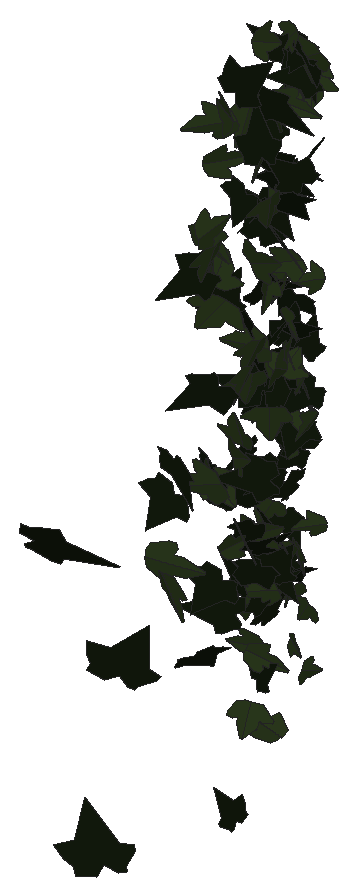
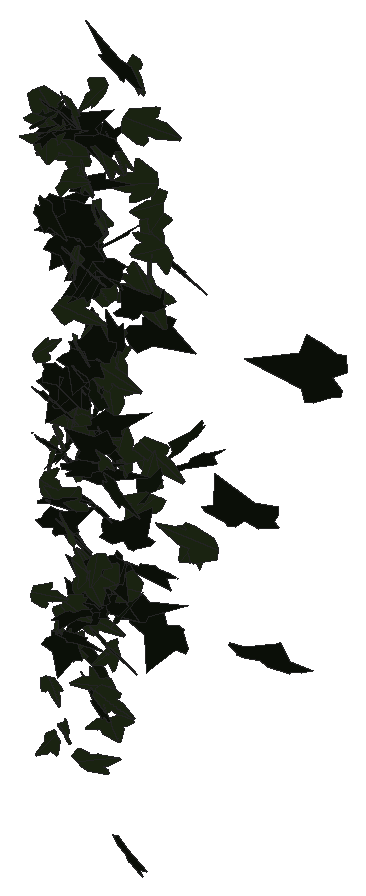
# SketchUp Ruby script. Lengths in inches.
U = 1.inch
M = Sketchup.active_model
def pt(a) = Geom::Point3d.new(a.map { |v| v * U })
def face(e, loops, mat)
  f = e.add_face(loops[0].map { |a| pt(a) })
  loops[1..].each { |l| e.add_face(l.map { |a| pt(a) }).erase! }
  f.material = f.back_material = mat if mat
  f
end
# faces: each face lists its corners as indices into pts; further lists are holes
def faces(e, pts, list, mat = nil) = list.each { |f| face(e, (f[0].is_a?(Array) ? f : [f]).map { |l| l.map { |i| pts[i] } }, mat) }
# xy, xz, yz: faces in a plane at the given z, y or x. An outline is a flat list of corners, or four numbers for a rectangle; further outlines are holes
def ring(l) = l.size == 4 ? [[l[0], l[1]], [l[2], l[1]], [l[2], l[3]], [l[0], l[3]]] : l.each_slice(2).to_a
def flat(e, list, mat, &to3) = list.each { |f| face(e, (f[0].is_a?(Array) ? f : [f]).map { |l| ring(l).map { |u, v| to3.(u, v) } }, mat) }
def xy(e, z, list, mat = nil) = flat(e, list, mat) { |x, y| [x, y, z] }
def xz(e, y, list, mat = nil) = flat(e, list, mat) { |x, z| [x, y, z] }
def yz(e, x, list, mat = nil) = flat(e, list, mat) { |y, z| [x, y, z] }
def lines(e, pts, list) = list.each { |a, b| e.add_line(pt(pts[a]), pt(pts[b])) }
# prism: a flat outline (further loops are holes) pulled along v
def prism(e, loops, v, mat = nil)
  f = face(e, loops, mat); d = Geom::Vector3d.new(v.map { |x| x * U })
  f.pushpull(f.normal.samedirection?(d) ? d.length : -d.length)
end
def box(e, o, s, mat = nil) = prism(e, [[o, [o[0] + s[0], o[1], o[2]], [o[0] + s[0], o[1] + s[1], o[2]], [o[0], o[1] + s[1], o[2]]]], [0, 0, s[2]], mat)
def at(x, y, z, deg = 0) = Geom::Transformation.translation(pt([x, y, z])) * Geom::Transformation.rotation(ORIGIN, Z_AXIS, deg.degrees)
def axes(o, x, y, z) = Geom::Transformation.new([*x, 0, *y, 0, *z, 0, *pt(o).to_a, 1])
def part(name) = M.definitions.add(name)
# library, detail: a bought-in or finely detailed component or shape, given as its bounding box
def library(name, o, s) = part(name).tap { |d| box(d.entities, o, s) }
def detail(e, o, s) = box(e.add_group.entities, o, s)
def put(e, d, t, mat = nil) = e.add_instance(d, t).tap { |i| i.material = mat if mat }
def group(e, t, mat = nil) = e.add_group.tap { |g| g.transformation = t; g.material = mat if mat }.entities
root = M.entities
M.materials.add("1026 AP 7946 SUNNY SIDE UP").color = [254, 231, 186]
M.materials.add("efeu1").color = [18, 25, 13]
M.materials.add("efeu2").color = [43, 57, 29]
c1 = part("ivyleaf_9")
p = [[1.54,2.16,1.25],[1.36,2.04,1.19],[-0.21,0.99,0.68],[-0.71,1.11,0.82],[-0.85,0.86,0.67],[-0.8,0.17,0.21],
  [-0.9,-0.01,0.1],[-0.67,-0.16,-0.02],[-0.08,-0.08,-0.05],[-0.03,-0.6,-0.4],[0.65,-0.88,-0.66],[0.83,-0.6,-0.49],
  [1.29,-0.42,-0.43],[1.8125,-0.07,-0.26],[1.21,0.44,0.15]]
faces(c1.entities,p,[[0,1,2,3,4,5,6,7,8,9,10,11,12,13,14]],"efeu1")
c2 = part("ivyleaf_10")
p = [[0,0.5,-0.03],[-0.0625,2.02,-0.43],[-0.19,2.01,-0.46],[-0.54,1.05,-0.29],[-0.52,0.625,-0.18],[-0.83,0.76,-0.28],
  [-1.16,0.64,-0.33],[-1.15,0.33,-0.24],[-0.77,-0.39,0.02],[-0.3,-0.51,0.16],[0.04,-0.48,0.23],[-0.02,2.01,-0.4375],
  [-0.06,2.01,-0.43],[0.04,-0.49,0.23],[0.67,-0.49,0.14],[1.38,0.36,-0.2],[1.375,0.51,-0.24],[0.81,0.65,-0.19],
  [0.62,0.59,-0.15],[0.6,1.09,-0.28],[0.5,1.23,-0.31]]
faces(c2.entities,p,[[0,1,2,3,4,5,6,7,8,9,10],[11,12,0,13,14,15,16,17,18,19,20]],"efeu2")
put(root,c1,axes([143.91,204.23,258.27],[0.4442,-0.05472,0.34587],[0.52307,-0.04862,-0.29654],[0.114,0.43631,0.01296]),"1026 AP 7946 SUNNY SIDE UP")
put(root,c1,axes([145.62,204.32,250.95],[-0.6745,-0.03704,0.05582],[0.07961,0.04334,0.44203],[-0.06609,0.43022,-0.03716]),"1026 AP 7946 SUNNY SIDE UP")
put(root,c1,axes([145.2,205.4375,254.96],[-0.43099,0.00527,0.31558],[0.47929,-0.0364,0.28143],[0.04816,0.40942,0.02338]),"1026 AP 7946 SUNNY SIDE UP")
put(root,c2,axes([144.47,208,255.81],[-0.41617,0.22329,-0.15177],[0.14377,-0.12113,-0.35602],[-0.39647,-0.27831,0.03021]),"1026 AP 7946 SUNNY SIDE UP")
put(root,c1,axes([144.38,208.25,257.83],[-0.24288,-0.27765,0.15078],[-0.09553,-0.13538,-0.32789],[0.48537,-0.16558,0.01091]),"1026 AP 7946 SUNNY SIDE UP")
put(root,c1,axes([145.43,208.44,260.77],[0.0087,0.02505,-0.3572],[-0.09637,-0.34142,-0.02841],[-0.53829,0.06153,-0.00069]),"1026 AP 7946 SUNNY SIDE UP")
put(root,c1,axes([144.24,208.49,258.49],[0.14987,-0.32445,0.08732],[0.03251,-0.08418,-0.34884],[0.52702,0.09746,-0.00331]),"1026 AP 7946 SUNNY SIDE UP")
put(root,c2,axes([143.93,208.34,256.05],[0.03397,-0.0484,-0.39616],[0.59854,-0.06837,0.03052],[-0.11239,-0.37876,0.04279]),"1026 AP 7946 SUNNY SIDE UP")
put(root,c2,axes([145.09,208.79,258.1],[-0.27734,0.02978,0.32535],[-0.49487,-0.06011,-0.17568],[0.06026,-0.35655,0.05463]),"1026 AP 7946 SUNNY SIDE UP")
put(root,c1,axes([144.78,208.55,253.875],[0.2302,0.31567,0.08074],[0.05949,0.06686,-0.35802],[-0.50728,0.15109,-0.00535]),"1026 AP 7946 SUNNY SIDE UP")
put(root,c2,axes([144.91,208.93,263.68],[0.00073,-0.39232,0.02905],[0.0109,-0.03041,-0.40428],[0.61863,0.001,0.00709]),"1026 AP 7946 SUNNY SIDE UP")
put(root,c1,axes([144.71,208.98,263.08],[-0.58845,0.09659,-0.02919],[0.02876,-0.04412,-0.3965],[-0.15589,-0.37275,0.03701]),"1026 AP 7946 SUNNY SIDE UP")
put(root,c1,axes([144.96,209.17,255.52],[-0.45271,-0.12464,-0.02536],[0.05178,-0.01612,-0.32203],[0.19272,-0.28845,0.02695]),"1026 AP 7946 SUNNY SIDE UP")
put(root,c2,axes([145.35,208.93,267.17],[0.05949,-0.05854,-0.35999],[-0.25234,0.3101,-0.06968],[0.49611,0.16475,0.00773]),"1026 AP 7946 SUNNY SIDE UP")
put(root,c2,axes([144.75,208.85,264.1],[0.03865,0.05038,-0.38805],[0.18583,0.35804,0.05933],[0.5684,-0.12048,0.00699]),"1026 AP 7946 SUNNY SIDE UP")
put(root,c2,axes([144.74,209.2,257.73],[-0.37546,0.20756,-0.02116],[-0.00703,0.02791,0.32557],[0.32808,0.23814,-0.01724]),"1026 AP 7946 SUNNY SIDE UP")
put(root,c2,axes([144.84,209.28,262.18],[0.51569,0.08418,-0.16296],[-0.2691,0.04622,-0.3389],[-0.0857,0.36138,0.08357]),"1026 AP 7946 SUNNY SIDE UP")
put(root,c1,axes([145.04,209.48,254.58],[-0.21895,-0.02923,0.30761],[-0.4295,-0.12425,-0.1444],[0.19576,-0.3053,0.02722]),"1026 AP 7946 SUNNY SIDE UP")
put(root,c2,axes([144.31,209.66,262.91],[-0.02449,0.05967,0.36681],[0.3821,-0.26139,0.0546],[0.41913,0.24178,-0.02834]),"1026 AP 7946 SUNNY SIDE UP")
put(root,c2,axes([145.34,209.58,260.57],[0.06103,-0.33213,0.12291],[0.04565,-0.11852,-0.34487],[0.55405,0.04635,0.01488]),"1026 AP 7946 SUNNY SIDE UP")
put(root,c2,axes([144.67,209.6875,266.47],[-0.1374,-0.08334,0.35157],[-0.32061,-0.27493,-0.12439],[0.45069,-0.22098,0.01869]),"1026 AP 7946 SUNNY SIDE UP")
put(root,c1,axes([144.26,209.76,257.83],[0.0974,-0.24531,0.18824],[0.06358,-0.17966,-0.26167],[0.47807,0.07387,-0.00355]),"1026 AP 7946 SUNNY SIDE UP")
put(root,c2,axes([144.14,209.625,263.62],[-0.35989,0.05646,-0.24104],[0.33274,-0.10756,-0.24029],[-0.18137,-0.30937,0.03747]),"1026 AP 7946 SUNNY SIDE UP")
put(root,c1,axes([145.09,209.58,267.42],[-0.19331,0.22963,0.3027],[0.26332,-0.24091,0.26591],[0.52212,0.20652,-0.02204]),"1026 AP 7946 SUNNY SIDE UP")
put(root,c1,axes([144.625,209.54,261.95],[-0.23618,-0.0729,0.29027],[0.39041,0.13422,0.17266],[-0.23996,0.29012,-0.00478]),"1026 AP 7946 SUNNY SIDE UP")
put(root,c2,axes([144.86,209.8,258.22],[-0.21327,0.10122,0.26268],[0.36849,-0.10391,0.17069],[0.22264,0.26893,-0.03088]),"1026 AP 7946 SUNNY SIDE UP")
put(root,c2,axes([144.48,209.64,262.59],[0.50208,-0.04558,-0.03787],[0.06494,0.03285,0.33014],[-0.06491,-0.3197,0.0374]),"1026 AP 7946 SUNNY SIDE UP")
put(root,c2,axes([145.41,209.83,261.17],[-0.04986,-0.34863,0.07419],[0.00198,-0.0744,-0.36099],[0.5604,-0.03076,0.00787]),"1026 AP 7946 SUNNY SIDE UP")
put(root,c1,axes([145.63,209.96,257.88],[-0.31775,-0.05214,0.25719],[-0.36035,-0.1035,-0.21373],[0.17702,-0.3043,0.02659]),"1026 AP 7946 SUNNY SIDE UP")
put(root,c2,axes([144.32,209.68,257.5625],[0.20932,0.25762,0.17923],[0.14155,0.14754,-0.29767],[-0.46651,0.16036,-0.0099]),"1026 AP 7946 SUNNY SIDE UP")
put(root,c2,axes([145.16,209.91,252.1],[0.32918,0.21096,-0.08231],[-0.06538,-0.0727,-0.30584],[-0.34931,0.21241,-0.02032]),"1026 AP 7946 SUNNY SIDE UP")
put(root,c2,axes([144.91,209.91,258.64],[-0.45055,0.09748,-0.03646],[-0.03966,0.03701,0.3108],[0.15847,0.2864,-0.02586]),"1026 AP 7946 SUNNY SIDE UP")
put(root,c2,axes([145.11,210.03,260.17],[-0.21876,-0.31771,-0.00263],[0.00896,-0.00168,-0.35727],[0.49949,-0.13912,0.00526]),"1026 AP 7946 SUNNY SIDE UP")
put(root,c2,axes([144.26,209.85,265.23],[0.03853,-0.07058,0.36115],[0.13044,0.34334,0.06717],[-0.54759,0.07682,0.04141]),"1026 AP 7946 SUNNY SIDE UP")
put(root,c1,axes([145.41,210.02,265.79],[-0.27882,-0.20444,0.27],[0.22964,0.22038,0.27894],[-0.47111,0.22842,-0.02383]),"1026 AP 7946 SUNNY SIDE UP")
put(root,c1,axes([144.65,210.35,261.39],[0.01829,-0.05422,0.30423],[0.09296,-0.28965,-0.05882],[0.46335,0.06025,-0.00021]),"1026 AP 7946 SUNNY SIDE UP")
put(root,c1,axes([144.53,210.25,256.8125],[0.22077,0.05238,0.2677],[-0.41191,-0.01538,0.14909],[0.06074,-0.2947,0.03802]),"1026 AP 7946 SUNNY SIDE UP")
put(root,c1,axes([144.72,210.23,254.875],[-0.03217,-0.25559,0.12409],[0.01082,0.12174,0.26485],[-0.44514,0.02143,-0.00253]),"1026 AP 7946 SUNNY SIDE UP")
put(root,c1,axes([144.67,210.03,249.17],[-0.05881,0.12042,0.27808],[-0.18278,0.24342,-0.12736],[-0.42625,-0.12099,0.01625]),"1026 AP 7946 SUNNY SIDE UP")
put(root,c1,axes([145.07,210.39,255.33],[0.02992,0.04935,-0.28548],[-0.07371,-0.2736,-0.05506],[-0.43685,0.04954,-0.01027]),"1026 AP 7946 SUNNY SIDE UP")
put(root,c1,axes([144.66,210.24,256.125],[0.33555,-0.11392,-0.1911],[-0.27399,0.0648,-0.24799],[0.20372,0.27479,-0.01877]),"1026 AP 7946 SUNNY SIDE UP")
put(root,c1,axes([145.01,210.4,252.57],[-0.06046,0.14227,0.23716],[0.11682,-0.21719,0.15032],[0.40806,0.08326,-0.0079]),"1026 AP 7946 SUNNY SIDE UP")
put(root,c2,axes([144.375,210.18,255.64],[-0.00582,-0.13898,0.26939],[0.06303,0.25967,0.14385],[-0.46247,0.03714,0.01622]),"1026 AP 7946 SUNNY SIDE UP")
put(root,c2,axes([145.07,210.39,260.78],[-0.12277,0.02895,0.35175],[-0.52892,-0.07238,-0.07338],[0.10139,-0.34253,0.04313]),"1026 AP 7946 SUNNY SIDE UP")
put(root,c1,axes([144.77,210.45,258.125],[-0.33274,0.15016,-0.12778],[0.12346,-0.1032,-0.26548],[-0.28119,-0.223,0.03465]),"1026 AP 7946 SUNNY SIDE UP")
put(root,c2,axes([144.97,210.32,253.2],[0.09614,0.04851,0.27505],[0.37204,0.1239,-0.07837],[-0.20805,0.24397,-0.01304]),"1026 AP 7946 SUNNY SIDE UP")
put(root,c2,axes([145.34,210.4,259.23],[-0.36009,-0.24597,-0.00627],[0.04484,-0.02018,-0.3445],[0.38423,-0.22816,0.03433]),"1026 AP 7946 SUNNY SIDE UP")
put(root,c2,axes([144.58,210.5,266.28],[0.44207,-0.2163,0.07976],[0.07273,-0.06853,-0.36489],[0.35452,0.28378,-0.0246]),"1026 AP 7946 SUNNY SIDE UP")
put(root,c2,axes([145.24,210.51,254.8],[-0.17451,-0.00987,0.26233],[-0.32796,-0.15615,-0.10078],[0.23036,-0.22979,0.05525]),"1026 AP 7946 SUNNY SIDE UP")
put(root,c1,axes([144.46,210.66,264.18],[-0.12344,-0.25181,0.14691],[-0.03493,-0.14356,-0.27187],[0.45481,-0.07937,0.01899]),"1026 AP 7946 SUNNY SIDE UP")
put(root,c1,axes([144.875,210.61,259.49],[-0.10681,0.00981,0.31975],[-0.44259,-0.13602,-0.05984],[0.20605,-0.28708,0.03722]),"1026 AP 7946 SUNNY SIDE UP")
put(root,c2,axes([144.83,210.53,262.67],[-0.3099,0.05947,0.29271],[0.44443,-0.03718,0.21002],[0.10174,0.34351,-0.02585]),"1026 AP 7946 SUNNY SIDE UP")
put(root,c2,axes([145.33,210.52,251.34],[0.17042,0.13198,0.23391],[-0.31625,-0.11501,0.16766],[0.26397,-0.22301,0.04986]),"1026 AP 7946 SUNNY SIDE UP")
put(root,c1,axes([144.84,210.5,256.23],[0.09736,0.17611,-0.21135],[-0.08379,-0.19943,-0.19317],[-0.41802,0.08099,-0.01051]),"1026 AP 7946 SUNNY SIDE UP")
put(root,c2,axes([145.23,210.5,264.33],[-0.09107,-0.35462,-0.06145],[0.03312,0.05493,-0.36965],[0.56395,-0.06049,0.01178]),"1026 AP 7946 SUNNY SIDE UP")
put(root,c1,axes([144.97,210.59,254.52],[-0.42206,0.14929,-0.03261],[0.02407,-0.0391,-0.31545],[-0.23903,-0.26754,0.02582]),"1026 AP 7946 SUNNY SIDE UP")
put(root,c1,axes([145.26,210.66,257.72],[-0.42536,0.03262,-0.06889],[0.09739,-0.04223,-0.27882],[-0.06529,-0.27548,0.03291]),"1026 AP 7946 SUNNY SIDE UP")
put(root,c1,axes([144.83,210.8125,260.05],[-0.05806,0.00026,0.32225],[-0.08682,-0.31003,-0.00826],[0.48412,-0.05557,0.03716]),"1026 AP 7946 SUNNY SIDE UP")
put(root,c2,axes([144.78,210.64,255.96],[-0.34347,-0.04192,0.22775],[0.34149,0.04258,0.22938],[-0.09395,0.30802,0.00115]),"1026 AP 7946 SUNNY SIDE UP")
put(root,c1,axes([144.79,210.57,255.61],[0.28361,0.24066,-0.01448],[-0.0092,0.02362,0.30936],[0.37908,-0.17948,0.01834]),"1026 AP 7946 SUNNY SIDE UP")
put(root,c1,axes([144.86,210.52,259.07],[-0.03731,0.09049,0.28187],[-0.16403,0.25267,-0.09411],[-0.42159,-0.10631,0.01167]),"1026 AP 7946 SUNNY SIDE UP")
put(root,c2,axes([144.75,210.67,253.18],[0.15918,-0.05165,-0.27939],[-0.39124,0.10736,-0.11625],[0.18704,0.26854,-0.00539]),"1026 AP 7946 SUNNY SIDE UP")
put(root,c2,axes([144.61,210.51,254.25],[-0.01221,-0.05394,-0.30535],[0.13119,0.2842,-0.05393],[0.4547,-0.08345,0.00736]),"1026 AP 7946 SUNNY SIDE UP")
put(root,c1,axes([145.16,210.6875,255.11],[-0.27465,0.08791,0.19696],[0.26677,-0.08705,0.20094],[0.19453,0.2435,0.00251]),"1026 AP 7946 SUNNY SIDE UP")
put(root,c1,axes([144.98,210.63,253.95],[-0.19247,0.27658,-0.0268],[-0.01222,0.02673,0.31172],[0.43688,0.1226,-0.00309]),"1026 AP 7946 SUNNY SIDE UP")
put(root,c2,axes([144.97,211.05,263.96],[-0.00437,0.0136,0.30235],[0.07949,-0.28902,0.0126],[0.45496,0.05063,0.0007]),"1026 AP 7946 SUNNY SIDE UP")
put(root,c2,axes([144.9,210.95,262.05],[0.00015,0.26309,-0.20274],[-0.04986,-0.19737,-0.27093],[-0.51562,0.01916,0.02614]),"1026 AP 7946 SUNNY SIDE UP")
put(root,c1,axes([144.8125,210.77,266.62],[0.00586,-0.02157,-0.35076],[0.38581,0.23657,-0.01129],[0.37244,-0.24472,0.01722]),"1026 AP 7946 SUNNY SIDE UP")
put(root,c1,axes([144.89,211.02,264.02],[-0.30432,0.22318,-0.19083],[0.14337,-0.16618,-0.3033],[-0.43428,-0.21125,0.0336]),"1026 AP 7946 SUNNY SIDE UP")
put(root,c2,axes([145.11,211.14,258.67],[0.01949,0.00659,0.27411],[0.21045,-0.23035,-0.00189],[0.36168,0.13368,-0.01367]),"1026 AP 7946 SUNNY SIDE UP")
put(root,c1,axes([145.03,210.91,255.07],[0.05629,-0.18958,-0.19092],[-0.02451,0.1841,-0.19719],[0.41497,0.03659,0.01425]),"1026 AP 7946 SUNNY SIDE UP")
put(root,c2,axes([145.22,210.78,260.13],[-0.01902,-0.17618,-0.2933],[0.04579,0.28225,-0.1802],[0.52311,-0.03111,0.00511]),"1026 AP 7946 SUNNY SIDE UP")
put(root,c1,axes([144.65,211.0625,256.15],[0.24381,-0.20665,0.07047],[0.03743,-0.06882,-0.26564],[0.34081,0.15539,-0.02123]),"1026 AP 7946 SUNNY SIDE UP")
put(root,c2,axes([144.38,211.08,266.34],[0.42145,-0.1183,0.0566],[0.06314,-0.04622,-0.30093],[0.1956,0.26981,-0.02481]),"1026 AP 7946 SUNNY SIDE UP")
put(root,c1,axes([144.61,211.09,261.54],[0.26174,0.18837,0.21342],[-0.23698,-0.14137,0.25769],[0.36959,-0.22405,0.01409]),"1026 AP 7946 SUNNY SIDE UP")
put(root,c1,axes([144.83,210.83,260.51],[-0.17504,0.25519,-0.07292],[-0.02999,0.07043,0.28704],[0.41594,0.11247,-0.00999]),"1026 AP 7946 SUNNY SIDE UP")
put(root,c2,axes([144.51,211.1875,264.99],[0.22361,-0.24269,0.15532],[0.09571,-0.14038,-0.29012],[0.44011,0.15384,-0.01582]),"1026 AP 7946 SUNNY SIDE UP")
put(root,c1,axes([145.55,211.18,264.65],[0.04415,0.06939,0.31023],[-0.43396,-0.12956,0.05658],[0.21729,-0.27285,0.04997]),"1026 AP 7946 SUNNY SIDE UP")
put(root,c1,axes([145.51,211.05,257.28],[-0.3017,0.22862,-0.03871],[0.02206,-0.03892,-0.30736],[-0.36397,-0.19186,0.01346]),"1026 AP 7946 SUNNY SIDE UP")
put(root,c1,axes([145.17,210.92,264.1875],[0.36845,0.22424,0.04542],[0.07357,0.01288,-0.33322],[-0.35134,0.23786,-0.02214]),"1026 AP 7946 SUNNY SIDE UP")
put(root,c2,axes([145.17,211.26,255.45],[-0.07262,-0.18695,0.19795],[-0.05613,-0.19004,-0.19933],[0.41899,-0.05786,0.0076]),"1026 AP 7946 SUNNY SIDE UP")
put(root,c1,axes([144.75,211.09,263.38],[0.47154,-0.19393,-0.09586],[-0.13831,0.03305,-0.36718],[0.30783,0.31192,-0.01814]),"1026 AP 7946 SUNNY SIDE UP")
put(root,c1,axes([144.625,210.97,263.12],[-0.14167,-0.02741,0.32879],[0.42671,0.16991,0.09491],[-0.26806,0.28496,-0.02269]),"1026 AP 7946 SUNNY SIDE UP")
put(root,c2,axes([145.15,211.33,254.51],[0.09874,-0.08801,0.22988],[0.18467,-0.19044,-0.11229],[0.32972,0.13302,-0.00595]),"1026 AP 7946 SUNNY SIDE UP")
put(root,c2,axes([145.08,211.32,260.38],[0.08033,-0.18666,-0.18995],[0.09302,-0.1737,0.19818],[-0.40073,-0.07774,0.00793]),"1026 AP 7946 SUNNY SIDE UP")
put(root,c1,axes([144.47,211.15,263.9],[-0.11946,-0.1463,-0.2863],[0.24585,0.22938,-0.16759],[0.42696,-0.17301,0.0164]),"1026 AP 7946 SUNNY SIDE UP")
put(root,c2,axes([145.25,211.27,262.55],[0.20593,0.03684,-0.28677],[-0.42576,-0.06562,-0.14047],[-0.11812,0.30075,0.00635]),"1026 AP 7946 SUNNY SIDE UP")
put(root,c1,axes([144.74,211.41,265.71],[-0.28344,-0.08501,0.24633],[-0.31454,-0.13384,-0.20475],[0.24671,-0.2683,0.02197]),"1026 AP 7946 SUNNY SIDE UP")
put(root,c2,axes([145.23,211.32,254.375],[-0.24041,-0.12217,-0.15773],[-0.18218,-0.0991,0.20099],[-0.24728,0.19179,0.00526]),"1026 AP 7946 SUNNY SIDE UP")
put(root,c2,axes([144.6,210.98,267.84],[-0.02496,0.12198,0.32132],[-0.07971,0.30708,-0.12486],[-0.51951,-0.05297,0.00372]),"1026 AP 7946 SUNNY SIDE UP")
put(root,c2,axes([144.97,211.41,261.04],[-0.11813,0.09192,-0.24533],[0.20657,-0.19955,-0.12295],[-0.34504,-0.15094,0.01038]),"1026 AP 7946 SUNNY SIDE UP")
put(root,c2,axes([144.59,211.37,256.29],[-0.30579,-0.14849,0.10176],[-0.0949,-0.08404,-0.25091],[0.26466,-0.20169,0.02761]),"1026 AP 7946 SUNNY SIDE UP")
put(root,c2,axes([145.0625,211.23,259.86],[0.34594,0.08814,-0.12978],[0.16522,0.07555,0.24297],[0.17738,-0.24227,0.02681]),"1026 AP 7946 SUNNY SIDE UP")
put(root,c1,axes([144.84,211.55,258.9375],[-0.2196,0.02231,0.27327],[-0.38834,-0.12226,-0.12414],[0.15563,-0.27359,0.07583]),"1026 AP 7946 SUNNY SIDE UP")
put(root,c2,axes([144.77,211.49,261.88],[0.29683,-0.22843,0.05507],[0.03207,-0.05403,-0.30501],[0.36796,0.18898,-0.01783]),"1026 AP 7946 SUNNY SIDE UP")
put(root,c1,axes([144.57,211.3,264.8],[0.40362,0.0497,0.17946],[0.27643,0.0025,-0.26802],[-0.06694,0.31005,-0.02474]),"1026 AP 7946 SUNNY SIDE UP")
put(root,c2,axes([144.34,211.4,256.87],[-0.06917,-0.25657,-0.07657],[0.09906,0.06177,-0.26287],[0.40752,-0.05856,0.0509]),"1026 AP 7946 SUNNY SIDE UP")
put(root,c2,axes([144.21,211.5,259.5],[0.36975,-0.08448,0.07848],[0.10182,-0.04574,-0.25683],[0.14768,0.24306,-0.01942]),"1026 AP 7946 SUNNY SIDE UP")
put(root,c2,axes([144.9,211.32,266.32],[0.06282,0.0661,0.32024],[0.39624,0.18369,-0.07262],[-0.30354,0.25348,-0.02852]),"1026 AP 7946 SUNNY SIDE UP")
put(root,c2,axes([144.86,211.29,265.93],[-0.03583,0.04746,0.32669],[-0.41617,0.17621,-0.04577],[-0.28388,-0.26431,0.02586]),"1026 AP 7946 SUNNY SIDE UP")
put(root,c1,axes([145.01,211.6,254.95],[-0.349,0.00441,0.10369],[-0.1581,-0.02381,-0.22755],[0.00917,-0.24253,0.02279]),"1026 AP 7946 SUNNY SIDE UP")
put(root,c2,axes([145.29,211.52,259.63],[0.20765,-0.26513,-0.07214],[-0.0583,0.05806,-0.30472],[0.42663,0.13698,-0.00653]),"1026 AP 7946 SUNNY SIDE UP")
put(root,c1,axes([145.52,211.625,259.38],[-0.45585,0.0138,-0.07349],[0.10784,-0.0458,-0.29623],[-0.03806,-0.29504,0.04078]),"1026 AP 7946 SUNNY SIDE UP")
put(root,c2,axes([144.97,211.42,260.23],[-0.25831,0.23625,0.11121],[-0.11262,0.07993,-0.2957],[-0.39168,-0.17879,0.01168]),"1026 AP 7946 SUNNY SIDE UP")
put(root,c1,axes([144.98,211.41,260.51],[-0.15953,-0.11723,0.27098],[0.29461,0.18584,0.16046],[-0.34513,0.21282,0.01171]),"1026 AP 7946 SUNNY SIDE UP")
put(root,c1,axes([145.02,211.38,260.76],[0.32344,0.22134,0.0364],[0.05702,0.01274,-0.31068],[-0.3475,0.20811,-0.0171]),"1026 AP 7946 SUNNY SIDE UP")
put(root,c1,axes([144.81,211.48,264.32],[0.34111,0.14837,-0.1646],[-0.19145,-0.10596,-0.27088],[-0.28559,0.24825,-0.01501]),"1026 AP 7946 SUNNY SIDE UP")
put(root,c2,axes([145.15,211.57,255.34],[-0.24295,0.20979,-0.07153],[0.04104,-0.06826,-0.26812],[-0.34564,-0.15557,0.01844]),"1026 AP 7946 SUNNY SIDE UP")
put(root,c1,axes([145.41,211.76,266.89],[-0.27913,-0.04165,0.24475],[-0.2875,-0.16958,-0.17219],[0.24793,-0.24354,0.07588]),"1026 AP 7946 SUNNY SIDE UP")
put(root,c1,axes([144.21,211.49,259.55],[-0.03854,-0.05171,0.26401],[0.38731,0.08256,0.04187],[-0.13912,0.24416,0.04342]),"1026 AP 7946 SUNNY SIDE UP")
put(root,c2,axes([145.39,211.78,258.53],[0.03983,-0.18564,0.21596],[0.04962,-0.20832,-0.19422],[0.43873,0.04041,0.00236]),"1026 AP 7946 SUNNY SIDE UP")
put(root,c2,axes([144.44,211.78,256.8125],[-0.09205,0.08472,-0.30534],[0.22083,-0.26178,-0.10703],[-0.4323,-0.15176,0.01035]),"1026 AP 7946 SUNNY SIDE UP")
put(root,c1,axes([145.02,211.82,258.28],[-0.28585,-0.22147,-0.01237],[0.07402,-0.02497,-0.29039],[0.34071,-0.18039,0.05271]),"1026 AP 7946 SUNNY SIDE UP")
put(root,c1,axes([145.4,211.5,260.26],[-0.37171,0.16706,0.02142],[0.04346,0.00481,0.29754],[0.26094,0.23718,-0.01904]),"1026 AP 7946 SUNNY SIDE UP")
put(root,c1,axes([145.08,211.73,257.66],[-0.41645,0.05459,-0.05864],[0.07801,-0.04112,-0.27714],[-0.09685,-0.26782,0.02893]),"1026 AP 7946 SUNNY SIDE UP")
put(root,c1,axes([144.52,211.54,261.63],[0.2622,0.18491,-0.02575],[-0.00841,-0.03017,-0.25615],[-0.2935,0.16606,-0.01566]),"1026 AP 7946 SUNNY SIDE UP")
put(root,c2,axes([145.63,211.63,267.61],[-0.32583,0.02429,0.23037],[-0.35293,-0.00553,-0.21382],[-0.01957,-0.30472,0.02045]),"1026 AP 7946 SUNNY SIDE UP")
put(root,c1,axes([144.88,211.69,259.55],[0.2399,-0.2271,-0.08683],[-0.09089,0.06104,-0.28116],[0.36917,0.1626,-0.0128]),"1026 AP 7946 SUNNY SIDE UP")
put(root,c1,axes([144.72,211.75,267.28],[0.04198,0.03954,0.28417],[-0.43726,-0.01026,0.02921],[0.02221,-0.27672,0.03786]),"1026 AP 7946 SUNNY SIDE UP")
put(root,c1,axes([145.06,211.54,254.69],[0.1353,0.22794,0.02881],[0.02371,0.0228,-0.25078],[-0.36007,0.08715,-0.00569]),"1026 AP 7946 SUNNY SIDE UP")
put(root,c2,axes([145.28,211.64,259.38],[-0.22411,0.25633,0.01582],[-0.03202,0.00456,-0.30169],[-0.40237,-0.14313,0.0152]),"1026 AP 7946 SUNNY SIDE UP")
put(root,c1,axes([145.17,211.83,267.56],[-0.42466,-0.00247,-0.10624],[0.16084,-0.04342,-0.27519],[-0.02077,-0.2858,0.04102]),"1026 AP 7946 SUNNY SIDE UP")
put(root,c2,axes([144.78,211.84,252.76],[0.02892,-0.00337,0.21416],[0.28253,-0.10478,-0.01874],[0.16453,0.18051,-0.00547]),"1026 AP 7946 SUNNY SIDE UP")
put(root,c2,axes([145.49,211.89,255.9],[-0.0561,-0.03528,0.232],[-0.16523,-0.19996,-0.05054],[0.31842,-0.10997,0.01465]),"1026 AP 7946 SUNNY SIDE UP")
put(root,c1,axes([145.2,211.96,267.42],[0.01956,-0.27485,0.14723],[0.05246,-0.14257,-0.28321],[0.48542,0.02648,0.02467]),"1026 AP 7946 SUNNY SIDE UP")
put(root,c1,axes([145.08,211.875,257.66],[0.01143,0.02724,0.28742],[-0.41978,-0.08393,0.01513],[0.13363,-0.26601,0.02293]),"1026 AP 7946 SUNNY SIDE UP")
put(root,c2,axes([144.84,211.76,267.81],[0.28025,-0.20868,-0.09866],[-0.11038,0.06433,-0.28212],[0.34294,0.19124,-0.01018]),"1026 AP 7946 SUNNY SIDE UP")
put(root,c2,axes([144.99,211.86,267.28],[-0.20748,0.13766,-0.20601],[0.19983,-0.1558,-0.19702],[-0.32645,-0.18286,0.01033]),"1026 AP 7946 SUNNY SIDE UP")
put(root,c2,axes([144.89,211.74,258.26],[0.40965,0.07036,0.11248],[-0.17638,0.00025,0.27657],[0.10193,-0.28232,0.02653]),"1026 AP 7946 SUNNY SIDE UP")
put(root,c1,axes([144.93,211.78,261.36],[0.20823,0.08522,-0.20942],[-0.23062,-0.14372,-0.16095],[-0.25968,0.19597,-0.02499]),"1026 AP 7946 SUNNY SIDE UP")
put(root,c2,axes([145.32,211.63,252.375],[-0.04487,-0.09902,-0.233],[0.11858,0.21271,-0.10476],[0.36882,-0.08043,0.00533]),"1026 AP 7946 SUNNY SIDE UP")
put(root,c2,axes([144.76,211.77,257.51],[0.27693,-0.21572,0.04964],[-0.01174,0.05731,0.28555],[-0.34778,-0.1737,0.02989]),"1026 AP 7946 SUNNY SIDE UP")
put(root,c2,axes([145.31,211.86,267.23],[0.45312,0.03374,-0.03449],[-0.04783,-0.02868,-0.29798],[-0.0577,0.28871,-0.02384]),"1026 AP 7946 SUNNY SIDE UP")
put(root,c1,axes([145.43,211.88,265.125],[-0.24151,0.16253,-0.17611],[0.15814,-0.14061,-0.2304],[-0.33666,-0.18264,0.01811]),"1026 AP 7946 SUNNY SIDE UP")
put(root,c2,axes([145.27,211.8,253.8125],[-0.28448,0.08225,0.11551],[-0.19137,-0.00619,-0.1985],[-0.10453,-0.21251,0.04906]),"1026 AP 7946 SUNNY SIDE UP")
put(root,c1,axes([144.92,212.05,267.17],[-0.26336,-0.22386,0.0476],[0.01356,-0.06497,-0.28462],[0.35957,-0.16151,0.0456]),"1026 AP 7946 SUNNY SIDE UP")
put(root,c2,axes([144.4375,212.04,264.25],[0.00959,0.11707,-0.25287],[-0.01782,-0.24587,-0.12221],[-0.42819,0.01286,-0.00058]),"1026 AP 7946 SUNNY SIDE UP")
put(root,c2,axes([144.59,211.76,264.29],[-0.20937,0.18934,0.12224],[-0.13354,0.08353,-0.23716],[-0.32402,-0.15677,0.01876]),"1026 AP 7946 SUNNY SIDE UP")
put(root,c2,axes([145.33,212.0625,261.79],[-0.06343,0.07061,0.26654],[0.03346,-0.25957,0.075],[0.41976,0.03136,0.0343]),"1026 AP 7946 SUNNY SIDE UP")
put(root,c2,axes([145.24,211.91,266.78],[0.46708,0.09334,0.03654],[0.06388,-0.01309,-0.31985],[-0.14311,0.29881,-0.0235]),"1026 AP 7946 SUNNY SIDE UP")
put(root,c2,axes([144.66,212.05,266.125],[0.09663,0.08876,-0.2609],[-0.19189,-0.22272,-0.11201],[-0.37665,0.13624,-0.00987]),"1026 AP 7946 SUNNY SIDE UP")
put(root,c1,axes([144.53,211.93,255.79],[-0.02577,-0.22724,-0.10568],[0.03696,0.09964,-0.23362],[0.38945,-0.02449,0.01518]),"1026 AP 7946 SUNNY SIDE UP")
put(root,c1,axes([144.7,211.87,264.28],[-0.31177,0.15363,0.05593],[-0.09045,0.01255,-0.25707],[-0.23923,-0.20496,0.0243]),"1026 AP 7946 SUNNY SIDE UP")
put(root,c1,axes([144.94,211.98,267.16],[0.0272,-0.30291,-0.0878],[-0.01924,0.08292,-0.31199],[0.49369,0.01992,-0.00732]),"1026 AP 7946 SUNNY SIDE UP")
